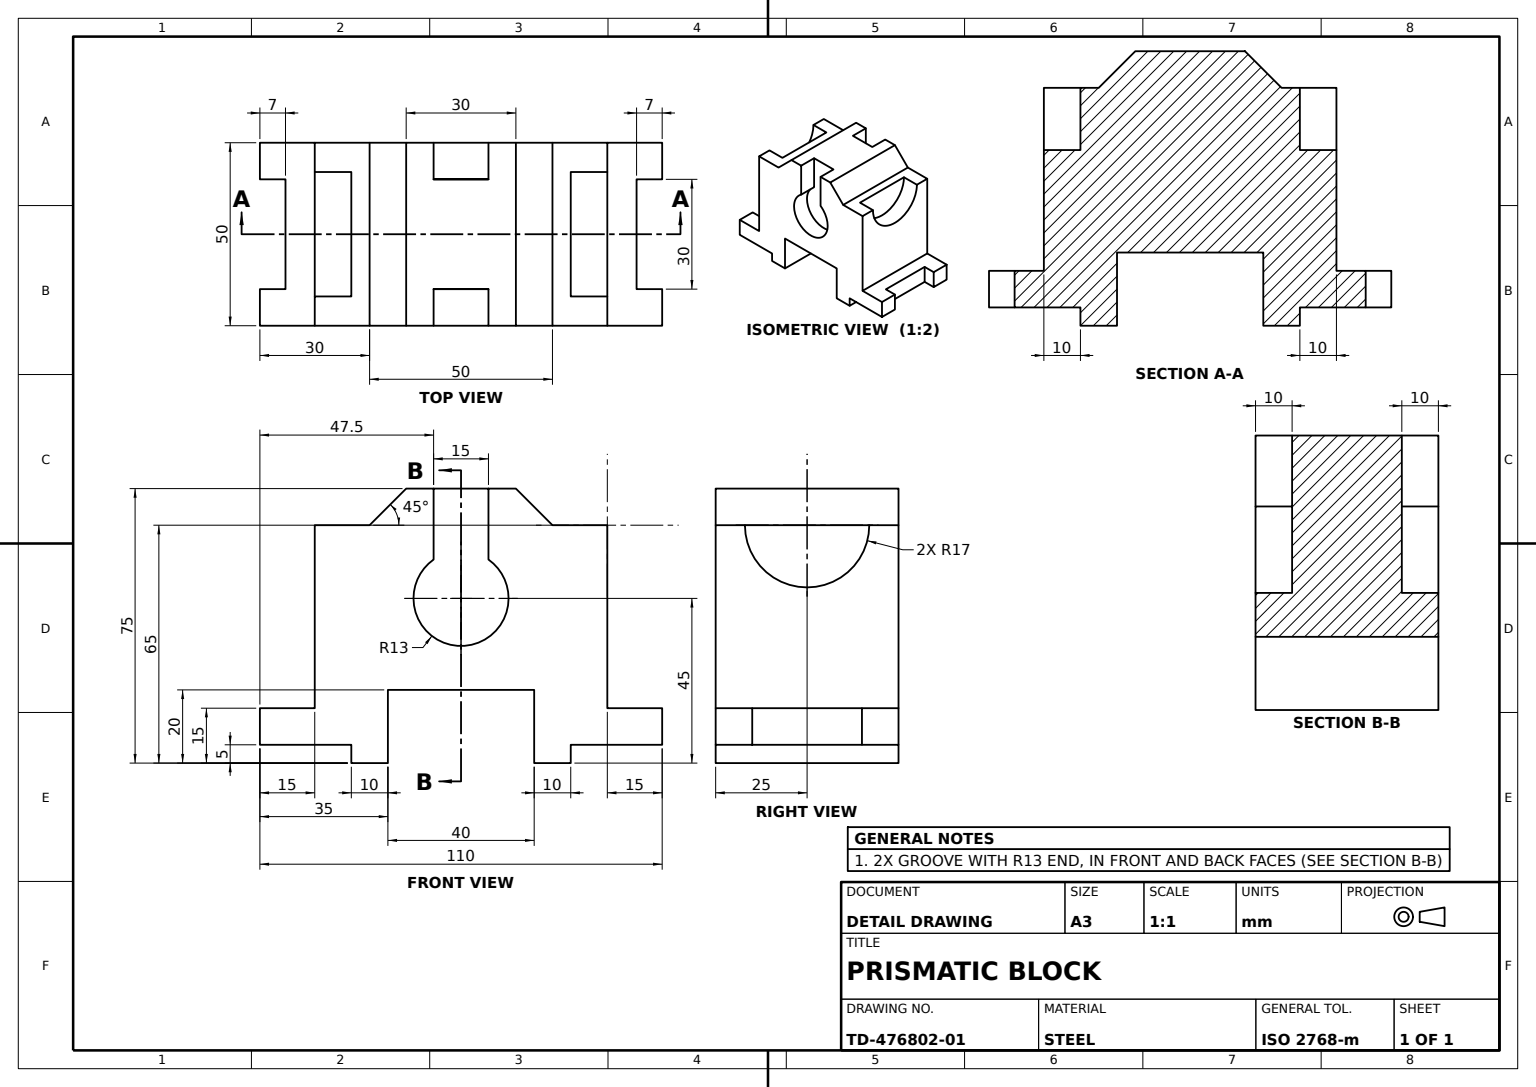
ISO-10303-21;
HEADER;
FILE_DESCRIPTION((''),'2;1');
FILE_NAME('','',(''),(''),'','','');
FILE_SCHEMA(('AUTOMOTIVE_DESIGN'));
ENDSEC;
DATA;
#1=APPLICATION_CONTEXT('');
#2=PRODUCT_CONTEXT('',#1,'mechanical');
#3=PRODUCT('','','',(#2));
#4=PRODUCT_DEFINITION_FORMATION('','',#3);
#5=PRODUCT_DEFINITION_CONTEXT('',#1,'design');
#6=PRODUCT_DEFINITION('','',#4,#5);
#7=PRODUCT_DEFINITION_SHAPE('','',#6);
#8=(LENGTH_UNIT()NAMED_UNIT(*)SI_UNIT(.MILLI.,.METRE.));
#9=(NAMED_UNIT(*)PLANE_ANGLE_UNIT()SI_UNIT($,.RADIAN.));
#10=(NAMED_UNIT(*)SI_UNIT($,.STERADIAN.)SOLID_ANGLE_UNIT());
#11=UNCERTAINTY_MEASURE_WITH_UNIT(LENGTH_MEASURE(1.E-05),#8,'distance_accuracy_value','');
#12=(GEOMETRIC_REPRESENTATION_CONTEXT(3)GLOBAL_UNCERTAINTY_ASSIGNED_CONTEXT((#11))GLOBAL_UNIT_ASSIGNED_CONTEXT((#8,#9,#10))REPRESENTATION_CONTEXT('',''));
#13=CARTESIAN_POINT('',(22.5,55.61838,0.));
#14=VERTEX_POINT('',#13);
#15=CARTESIAN_POINT('',(22.5,75.,0.));
#16=VERTEX_POINT('',#15);
#17=DIRECTION('',(0.,1.,0.));
#18=VECTOR('',#17,1000.);
#19=LINE('',#15,#18);
#20=EDGE_CURVE('',#14,#16,#19,.T.);
#21=ORIENTED_EDGE('',*,*,#20,.T.);
#22=CARTESIAN_POINT('',(22.5,75.,10.));
#23=VERTEX_POINT('',#22);
#24=DIRECTION('',(0.,0.,-1.));
#25=VECTOR('',#24,1000.);
#26=LINE('',#22,#25);
#27=EDGE_CURVE('',#23,#16,#26,.T.);
#28=ORIENTED_EDGE('',*,*,#27,.F.);
#29=CARTESIAN_POINT('',(22.5,55.61838,10.));
#30=VERTEX_POINT('',#29);
#31=LINE('',#22,#18);
#32=EDGE_CURVE('',#30,#23,#31,.T.);
#33=ORIENTED_EDGE('',*,*,#32,.F.);
#34=LINE('',#29,#25);
#35=EDGE_CURVE('',#30,#14,#34,.T.);
#36=ORIENTED_EDGE('',*,*,#35,.T.);
#37=EDGE_LOOP('',(#21,#28,#33,#36));
#38=FACE_OUTER_BOUND('',#37,.T.);
#39=DIRECTION('',(-1.,0.,0.));
#40=DIRECTION('',(0.,0.,1.));
#41=AXIS2_PLACEMENT_3D('',#22,#39,#40);
#42=PLANE('',#41);
#43=ADVANCED_FACE('',(#38),#42,.F.);
#44=CARTESIAN_POINT('',(0.,65.,8.));
#45=VERTEX_POINT('',#44);
#46=CARTESIAN_POINT('',(0.,65.,42.));
#47=VERTEX_POINT('',#46);
#48=CARTESIAN_POINT('',(0.,65.,25.));
#49=AXIS2_PLACEMENT_3D('',#48,#39,#40);
#50=CIRCLE('',#49,17.);
#51=EDGE_CURVE('',#45,#47,#50,.T.);
#52=ORIENTED_EDGE('',*,*,#51,.T.);
#53=LINE('',#44,#25);
#54=EDGE_CURVE('',#47,#45,#53,.T.);
#55=ORIENTED_EDGE('',*,*,#54,.T.);
#56=EDGE_LOOP('',(#52,#55));
#57=FACE_OUTER_BOUND('',#56,.T.);
#58=PLANE('',#49);
#59=ADVANCED_FACE('',(#57),#58,.T.);
#60=CARTESIAN_POINT('',(22.5,75.,50.));
#61=VERTEX_POINT('',#60);
#62=CARTESIAN_POINT('',(22.5,55.61838,50.));
#63=VERTEX_POINT('',#62);
#64=DIRECTION('',(0.,-1.,0.));
#65=VECTOR('',#64,1000.);
#66=LINE('',#60,#65);
#67=EDGE_CURVE('',#61,#63,#66,.T.);
#68=ORIENTED_EDGE('',*,*,#67,.T.);
#69=CARTESIAN_POINT('',(22.5,55.61838,40.));
#70=VERTEX_POINT('',#69);
#71=VECTOR('',#40,1000.);
#72=LINE('',#69,#71);
#73=EDGE_CURVE('',#70,#63,#72,.T.);
#74=ORIENTED_EDGE('',*,*,#73,.F.);
#75=CARTESIAN_POINT('',(22.5,75.,40.));
#76=VERTEX_POINT('',#75);
#77=LINE('',#75,#65);
#78=EDGE_CURVE('',#76,#70,#77,.T.);
#79=ORIENTED_EDGE('',*,*,#78,.F.);
#80=LINE('',#75,#71);
#81=EDGE_CURVE('',#76,#61,#80,.T.);
#82=ORIENTED_EDGE('',*,*,#81,.T.);
#83=EDGE_LOOP('',(#68,#74,#79,#82));
#84=FACE_OUTER_BOUND('',#83,.T.);
#85=AXIS2_PLACEMENT_3D('',#75,#39,#40);
#86=PLANE('',#85);
#87=ADVANCED_FACE('',(#84),#86,.F.);
#88=CARTESIAN_POINT('',(85.,5.,40.));
#89=VERTEX_POINT('',#88);
#90=CARTESIAN_POINT('',(85.,15.,40.));
#91=VERTEX_POINT('',#90);
#92=LINE('',#88,#18);
#93=EDGE_CURVE('',#89,#91,#92,.T.);
#94=ORIENTED_EDGE('',*,*,#93,.F.);
#95=CARTESIAN_POINT('',(78.,5.,40.));
#96=VERTEX_POINT('',#95);
#97=DIRECTION('',(1.,0.,0.));
#98=VECTOR('',#97,1000.);
#99=LINE('',#95,#98);
#100=EDGE_CURVE('',#96,#89,#99,.T.);
#101=ORIENTED_EDGE('',*,*,#100,.F.);
#102=CARTESIAN_POINT('',(78.,15.,40.));
#103=VERTEX_POINT('',#102);
#104=LINE('',#95,#18);
#105=EDGE_CURVE('',#96,#103,#104,.T.);
#106=ORIENTED_EDGE('',*,*,#105,.T.);
#107=LINE('',#102,#98);
#108=EDGE_CURVE('',#103,#91,#107,.T.);
#109=ORIENTED_EDGE('',*,*,#108,.T.);
#110=EDGE_LOOP('',(#94,#101,#106,#109));
#111=FACE_OUTER_BOUND('',#110,.T.);
#112=AXIS2_PLACEMENT_3D('',#95,#40,#97);
#113=PLANE('',#112);
#114=ADVANCED_FACE('',(#111),#113,.F.);
#115=CARTESIAN_POINT('',(-10.,65.,8.));
#116=VERTEX_POINT('',#115);
#117=CARTESIAN_POINT('',(-10.,65.,42.));
#118=VERTEX_POINT('',#117);
#119=CARTESIAN_POINT('',(-10.,65.,25.));
#120=AXIS2_PLACEMENT_3D('',#119,#39,#40);
#121=CIRCLE('',#120,17.);
#122=EDGE_CURVE('',#116,#118,#121,.T.);
#123=ORIENTED_EDGE('',*,*,#122,.T.);
#124=VECTOR('',#39,1000.);
#125=LINE('',#46,#124);
#126=EDGE_CURVE('',#47,#118,#125,.T.);
#127=ORIENTED_EDGE('',*,*,#126,.F.);
#128=ORIENTED_EDGE('',*,*,#51,.F.);
#129=LINE('',#44,#124);
#130=EDGE_CURVE('',#45,#116,#129,.T.);
#131=ORIENTED_EDGE('',*,*,#130,.T.);
#132=EDGE_LOOP('',(#123,#127,#128,#131));
#133=FACE_OUTER_BOUND('',#132,.T.);
#134=CYLINDRICAL_SURFACE('',#49,17.);
#135=ADVANCED_FACE('',(#133),#134,.F.);
#136=CARTESIAN_POINT('',(55.,65.,50.));
#137=VERTEX_POINT('',#136);
#138=CARTESIAN_POINT('',(45.,75.,50.));
#139=VERTEX_POINT('',#138);
#140=DIRECTION('',(-0.707106781,0.707106781,0.));
#141=VECTOR('',#140,1000.);
#142=LINE('',#138,#141);
#143=EDGE_CURVE('',#137,#139,#142,.T.);
#144=ORIENTED_EDGE('',*,*,#143,.F.);
#145=CARTESIAN_POINT('',(55.,65.,0.));
#146=VERTEX_POINT('',#145);
#147=LINE('',#136,#25);
#148=EDGE_CURVE('',#137,#146,#147,.T.);
#149=ORIENTED_EDGE('',*,*,#148,.T.);
#150=CARTESIAN_POINT('',(45.,75.,0.));
#151=VERTEX_POINT('',#150);
#152=LINE('',#150,#141);
#153=EDGE_CURVE('',#146,#151,#152,.T.);
#154=ORIENTED_EDGE('',*,*,#153,.T.);
#155=LINE('',#138,#25);
#156=EDGE_CURVE('',#139,#151,#155,.T.);
#157=ORIENTED_EDGE('',*,*,#156,.F.);
#158=EDGE_LOOP('',(#144,#149,#154,#157));
#159=FACE_OUTER_BOUND('',#158,.T.);
#160=DIRECTION('',(-0.707106781,-0.707106781,0.));
#161=DIRECTION('',(0.707106781,-0.707106781,0.));
#162=AXIS2_PLACEMENT_3D('',#138,#160,#161);
#163=PLANE('',#162);
#164=ADVANCED_FACE('',(#159),#163,.F.);
#165=CARTESIAN_POINT('',(60.,65.,42.));
#166=VERTEX_POINT('',#165);
#167=CARTESIAN_POINT('',(60.,65.,8.));
#168=VERTEX_POINT('',#167);
#169=CARTESIAN_POINT('',(60.,65.,25.));
#170=AXIS2_PLACEMENT_3D('',#169,#97,#24);
#171=CIRCLE('',#170,17.);
#172=EDGE_CURVE('',#166,#168,#171,.T.);
#173=ORIENTED_EDGE('',*,*,#172,.T.);
#174=LINE('',#165,#71);
#175=EDGE_CURVE('',#168,#166,#174,.T.);
#176=ORIENTED_EDGE('',*,*,#175,.T.);
#177=EDGE_LOOP('',(#173,#176));
#178=FACE_OUTER_BOUND('',#177,.T.);
#179=PLANE('',#170);
#180=ADVANCED_FACE('',(#178),#179,.T.);
#181=CARTESIAN_POINT('',(0.,0.,50.));
#182=VERTEX_POINT('',#181);
#183=CARTESIAN_POINT('',(0.,0.,0.));
#184=VERTEX_POINT('',#183);
#185=LINE('',#181,#25);
#186=EDGE_CURVE('',#182,#184,#185,.T.);
#187=ORIENTED_EDGE('',*,*,#186,.T.);
#188=CARTESIAN_POINT('',(10.,0.,0.));
#189=VERTEX_POINT('',#188);
#190=LINE('',#183,#98);
#191=EDGE_CURVE('',#184,#189,#190,.T.);
#192=ORIENTED_EDGE('',*,*,#191,.T.);
#193=CARTESIAN_POINT('',(10.,0.,50.));
#194=VERTEX_POINT('',#193);
#195=LINE('',#193,#25);
#196=EDGE_CURVE('',#194,#189,#195,.T.);
#197=ORIENTED_EDGE('',*,*,#196,.F.);
#198=LINE('',#181,#98);
#199=EDGE_CURVE('',#182,#194,#198,.T.);
#200=ORIENTED_EDGE('',*,*,#199,.F.);
#201=EDGE_LOOP('',(#187,#192,#197,#200));
#202=FACE_OUTER_BOUND('',#201,.T.);
#203=AXIS2_PLACEMENT_3D('',#181,#17,#40);
#204=PLANE('',#203);
#205=ADVANCED_FACE('',(#202),#204,.F.);
#206=CARTESIAN_POINT('',(37.5,75.,10.));
#207=VERTEX_POINT('',#206);
#208=CARTESIAN_POINT('',(30.,75.,10.));
#209=LINE('',#208,#98);
#210=EDGE_CURVE('',#23,#207,#209,.T.);
#211=ORIENTED_EDGE('',*,*,#210,.T.);
#212=CARTESIAN_POINT('',(37.5,55.61838,10.));
#213=VERTEX_POINT('',#212);
#214=LINE('',#206,#65);
#215=EDGE_CURVE('',#207,#213,#214,.T.);
#216=ORIENTED_EDGE('',*,*,#215,.T.);
#217=CARTESIAN_POINT('',(43.,45.,10.));
#218=VERTEX_POINT('',#217);
#219=CARTESIAN_POINT('',(30.,45.,10.));
#220=AXIS2_PLACEMENT_3D('',#219,#24,#39);
#221=CIRCLE('',#220,13.);
#222=EDGE_CURVE('',#213,#218,#221,.T.);
#223=ORIENTED_EDGE('',*,*,#222,.T.);
#224=CARTESIAN_POINT('',(17.,45.,10.));
#225=VERTEX_POINT('',#224);
#226=EDGE_CURVE('',#218,#225,#221,.T.);
#227=ORIENTED_EDGE('',*,*,#226,.T.);
#228=EDGE_CURVE('',#225,#30,#221,.T.);
#229=ORIENTED_EDGE('',*,*,#228,.T.);
#230=ORIENTED_EDGE('',*,*,#32,.T.);
#231=EDGE_LOOP('',(#211,#216,#223,#227,#229,#230));
#232=FACE_OUTER_BOUND('',#231,.T.);
#233=PLANE('',#220);
#234=ADVANCED_FACE('',(#232),#233,.T.);
#235=CARTESIAN_POINT('',(17.,45.,0.));
#236=VERTEX_POINT('',#235);
#237=CARTESIAN_POINT('',(30.,45.,0.));
#238=AXIS2_PLACEMENT_3D('',#237,#24,#39);
#239=CIRCLE('',#238,13.);
#240=EDGE_CURVE('',#236,#14,#239,.T.);
#241=ORIENTED_EDGE('',*,*,#240,.T.);
#242=ORIENTED_EDGE('',*,*,#35,.F.);
#243=ORIENTED_EDGE('',*,*,#228,.F.);
#244=LINE('',#224,#25);
#245=EDGE_CURVE('',#225,#236,#244,.T.);
#246=ORIENTED_EDGE('',*,*,#245,.T.);
#247=EDGE_LOOP('',(#241,#242,#243,#246));
#248=FACE_OUTER_BOUND('',#247,.T.);
#249=CYLINDRICAL_SURFACE('',#220,13.);
#250=ADVANCED_FACE('',(#248),#249,.F.);
#251=CARTESIAN_POINT('',(15.,75.,50.));
#252=VERTEX_POINT('',#251);
#253=CARTESIAN_POINT('',(5.,65.,50.));
#254=VERTEX_POINT('',#253);
#255=VECTOR('',#160,1000.);
#256=LINE('',#251,#255);
#257=EDGE_CURVE('',#252,#254,#256,.T.);
#258=ORIENTED_EDGE('',*,*,#257,.F.);
#259=CARTESIAN_POINT('',(15.,75.,0.));
#260=VERTEX_POINT('',#259);
#261=LINE('',#251,#25);
#262=EDGE_CURVE('',#252,#260,#261,.T.);
#263=ORIENTED_EDGE('',*,*,#262,.T.);
#264=CARTESIAN_POINT('',(5.,65.,0.));
#265=VERTEX_POINT('',#264);
#266=LINE('',#259,#255);
#267=EDGE_CURVE('',#260,#265,#266,.T.);
#268=ORIENTED_EDGE('',*,*,#267,.T.);
#269=LINE('',#253,#25);
#270=EDGE_CURVE('',#254,#265,#269,.T.);
#271=ORIENTED_EDGE('',*,*,#270,.F.);
#272=EDGE_LOOP('',(#258,#263,#268,#271));
#273=FACE_OUTER_BOUND('',#272,.T.);
#274=DIRECTION('',(0.707106781,0.707106781,0.));
#275=AXIS2_PLACEMENT_3D('',#251,#161,#274);
#276=PLANE('',#275);
#277=ADVANCED_FACE('',(#273),#276,.F.);
#278=CARTESIAN_POINT('',(50.,20.,50.));
#279=VERTEX_POINT('',#278);
#280=CARTESIAN_POINT('',(50.,20.,0.));
#281=VERTEX_POINT('',#280);
#282=LINE('',#278,#25);
#283=EDGE_CURVE('',#279,#281,#282,.T.);
#284=ORIENTED_EDGE('',*,*,#283,.F.);
#285=CARTESIAN_POINT('',(10.,20.,50.));
#286=VERTEX_POINT('',#285);
#287=LINE('',#285,#98);
#288=EDGE_CURVE('',#286,#279,#287,.T.);
#289=ORIENTED_EDGE('',*,*,#288,.F.);
#290=CARTESIAN_POINT('',(10.,20.,0.));
#291=VERTEX_POINT('',#290);
#292=LINE('',#285,#25);
#293=EDGE_CURVE('',#286,#291,#292,.T.);
#294=ORIENTED_EDGE('',*,*,#293,.T.);
#295=LINE('',#290,#98);
#296=EDGE_CURVE('',#291,#281,#295,.T.);
#297=ORIENTED_EDGE('',*,*,#296,.T.);
#298=EDGE_LOOP('',(#284,#289,#294,#297));
#299=FACE_OUTER_BOUND('',#298,.T.);
#300=AXIS2_PLACEMENT_3D('',#285,#17,#40);
#301=PLANE('',#300);
#302=ADVANCED_FACE('',(#299),#301,.F.);
#303=CARTESIAN_POINT('',(78.,5.,10.));
#304=VERTEX_POINT('',#303);
#305=CARTESIAN_POINT('',(78.,15.,10.));
#306=VERTEX_POINT('',#305);
#307=LINE('',#303,#18);
#308=EDGE_CURVE('',#304,#306,#307,.T.);
#309=ORIENTED_EDGE('',*,*,#308,.T.);
#310=LINE('',#305,#71);
#311=EDGE_CURVE('',#306,#103,#310,.T.);
#312=ORIENTED_EDGE('',*,*,#311,.T.);
#313=ORIENTED_EDGE('',*,*,#105,.F.);
#314=LINE('',#303,#71);
#315=EDGE_CURVE('',#304,#96,#314,.T.);
#316=ORIENTED_EDGE('',*,*,#315,.F.);
#317=EDGE_LOOP('',(#309,#312,#313,#316));
#318=FACE_OUTER_BOUND('',#317,.T.);
#319=AXIS2_PLACEMENT_3D('',#303,#39,#40);
#320=PLANE('',#319);
#321=ADVANCED_FACE('',(#318),#320,.F.);
#322=CARTESIAN_POINT('',(50.,0.,0.));
#323=VERTEX_POINT('',#322);
#324=LINE('',#280,#65);
#325=EDGE_CURVE('',#281,#323,#324,.T.);
#326=ORIENTED_EDGE('',*,*,#325,.T.);
#327=CARTESIAN_POINT('',(50.,0.,50.));
#328=VERTEX_POINT('',#327);
#329=LINE('',#327,#25);
#330=EDGE_CURVE('',#328,#323,#329,.T.);
#331=ORIENTED_EDGE('',*,*,#330,.F.);
#332=LINE('',#278,#65);
#333=EDGE_CURVE('',#279,#328,#332,.T.);
#334=ORIENTED_EDGE('',*,*,#333,.F.);
#335=ORIENTED_EDGE('',*,*,#283,.T.);
#336=EDGE_LOOP('',(#326,#331,#334,#335));
#337=FACE_OUTER_BOUND('',#336,.T.);
#338=AXIS2_PLACEMENT_3D('',#278,#97,#24);
#339=PLANE('',#338);
#340=ADVANCED_FACE('',(#337),#339,.F.);
#341=CARTESIAN_POINT('',(-18.,5.,10.));
#342=VERTEX_POINT('',#341);
#343=CARTESIAN_POINT('',(-25.,5.,10.));
#344=VERTEX_POINT('',#343);
#345=LINE('',#341,#124);
#346=EDGE_CURVE('',#342,#344,#345,.T.);
#347=ORIENTED_EDGE('',*,*,#346,.F.);
#348=CARTESIAN_POINT('',(-18.,15.,10.));
#349=VERTEX_POINT('',#348);
#350=LINE('',#341,#18);
#351=EDGE_CURVE('',#342,#349,#350,.T.);
#352=ORIENTED_EDGE('',*,*,#351,.T.);
#353=CARTESIAN_POINT('',(-25.,15.,10.));
#354=VERTEX_POINT('',#353);
#355=LINE('',#348,#124);
#356=EDGE_CURVE('',#349,#354,#355,.T.);
#357=ORIENTED_EDGE('',*,*,#356,.T.);
#358=LINE('',#343,#18);
#359=EDGE_CURVE('',#344,#354,#358,.T.);
#360=ORIENTED_EDGE('',*,*,#359,.F.);
#361=EDGE_LOOP('',(#347,#352,#357,#360));
#362=FACE_OUTER_BOUND('',#361,.T.);
#363=AXIS2_PLACEMENT_3D('',#341,#24,#39);
#364=PLANE('',#363);
#365=ADVANCED_FACE('',(#362),#364,.F.);
#366=ORIENTED_EDGE('',*,*,#186,.F.);
#367=CARTESIAN_POINT('',(0.,5.,50.));
#368=VERTEX_POINT('',#367);
#369=LINE('',#181,#65);
#370=EDGE_CURVE('',#368,#182,#369,.T.);
#371=ORIENTED_EDGE('',*,*,#370,.F.);
#372=CARTESIAN_POINT('',(0.,5.,0.));
#373=VERTEX_POINT('',#372);
#374=LINE('',#367,#25);
#375=EDGE_CURVE('',#368,#373,#374,.T.);
#376=ORIENTED_EDGE('',*,*,#375,.T.);
#377=LINE('',#183,#65);
#378=EDGE_CURVE('',#373,#184,#377,.T.);
#379=ORIENTED_EDGE('',*,*,#378,.T.);
#380=EDGE_LOOP('',(#366,#371,#376,#379));
#381=FACE_OUTER_BOUND('',#380,.T.);
#382=AXIS2_PLACEMENT_3D('',#181,#97,#24);
#383=PLANE('',#382);
#384=ADVANCED_FACE('',(#381),#383,.F.);
#385=CARTESIAN_POINT('',(17.,45.,40.));
#386=VERTEX_POINT('',#385);
#387=CARTESIAN_POINT('',(17.,45.,50.));
#388=VERTEX_POINT('',#387);
#389=LINE('',#385,#71);
#390=EDGE_CURVE('',#386,#388,#389,.T.);
#391=ORIENTED_EDGE('',*,*,#390,.F.);
#392=CARTESIAN_POINT('',(30.,45.,40.));
#393=AXIS2_PLACEMENT_3D('',#392,#40,#97);
#394=CIRCLE('',#393,13.);
#395=EDGE_CURVE('',#70,#386,#394,.T.);
#396=ORIENTED_EDGE('',*,*,#395,.F.);
#397=ORIENTED_EDGE('',*,*,#73,.T.);
#398=CARTESIAN_POINT('',(30.,45.,50.));
#399=AXIS2_PLACEMENT_3D('',#398,#40,#97);
#400=CIRCLE('',#399,13.);
#401=EDGE_CURVE('',#63,#388,#400,.T.);
#402=ORIENTED_EDGE('',*,*,#401,.T.);
#403=EDGE_LOOP('',(#391,#396,#397,#402));
#404=FACE_OUTER_BOUND('',#403,.T.);
#405=CYLINDRICAL_SURFACE('',#393,13.);
#406=ADVANCED_FACE('',(#404),#405,.F.);
#407=CARTESIAN_POINT('',(-25.,5.,40.));
#408=VERTEX_POINT('',#407);
#409=CARTESIAN_POINT('',(-18.,5.,40.));
#410=VERTEX_POINT('',#409);
#411=LINE('',#407,#98);
#412=EDGE_CURVE('',#408,#410,#411,.T.);
#413=ORIENTED_EDGE('',*,*,#412,.T.);
#414=LINE('',#409,#25);
#415=EDGE_CURVE('',#410,#342,#414,.T.);
#416=ORIENTED_EDGE('',*,*,#415,.T.);
#417=ORIENTED_EDGE('',*,*,#346,.T.);
#418=CARTESIAN_POINT('',(-25.,5.,0.));
#419=VERTEX_POINT('',#418);
#420=CARTESIAN_POINT('',(-25.,5.,50.));
#421=LINE('',#420,#25);
#422=EDGE_CURVE('',#344,#419,#421,.T.);
#423=ORIENTED_EDGE('',*,*,#422,.T.);
#424=LINE('',#372,#98);
#425=EDGE_CURVE('',#419,#373,#424,.T.);
#426=ORIENTED_EDGE('',*,*,#425,.T.);
#427=ORIENTED_EDGE('',*,*,#375,.F.);
#428=VERTEX_POINT('',#420);
#429=LINE('',#367,#98);
#430=EDGE_CURVE('',#428,#368,#429,.T.);
#431=ORIENTED_EDGE('',*,*,#430,.F.);
#432=EDGE_CURVE('',#428,#408,#421,.T.);
#433=ORIENTED_EDGE('',*,*,#432,.T.);
#434=EDGE_LOOP('',(#413,#416,#417,#423,#426,#427,#431,#433));
#435=FACE_OUTER_BOUND('',#434,.T.);
#436=AXIS2_PLACEMENT_3D('',#367,#17,#40);
#437=PLANE('',#436);
#438=ADVANCED_FACE('',(#435),#437,.F.);
#439=ORIENTED_EDGE('',*,*,#315,.T.);
#440=ORIENTED_EDGE('',*,*,#100,.T.);
#441=CARTESIAN_POINT('',(85.,5.,50.));
#442=VERTEX_POINT('',#441);
#443=LINE('',#441,#25);
#444=EDGE_CURVE('',#442,#89,#443,.T.);
#445=ORIENTED_EDGE('',*,*,#444,.F.);
#446=CARTESIAN_POINT('',(60.,5.,50.));
#447=VERTEX_POINT('',#446);
#448=LINE('',#446,#98);
#449=EDGE_CURVE('',#447,#442,#448,.T.);
#450=ORIENTED_EDGE('',*,*,#449,.F.);
#451=CARTESIAN_POINT('',(60.,5.,0.));
#452=VERTEX_POINT('',#451);
#453=LINE('',#446,#25);
#454=EDGE_CURVE('',#447,#452,#453,.T.);
#455=ORIENTED_EDGE('',*,*,#454,.T.);
#456=CARTESIAN_POINT('',(85.,5.,0.));
#457=VERTEX_POINT('',#456);
#458=LINE('',#451,#98);
#459=EDGE_CURVE('',#452,#457,#458,.T.);
#460=ORIENTED_EDGE('',*,*,#459,.T.);
#461=CARTESIAN_POINT('',(85.,5.,10.));
#462=VERTEX_POINT('',#461);
#463=EDGE_CURVE('',#462,#457,#443,.T.);
#464=ORIENTED_EDGE('',*,*,#463,.F.);
#465=LINE('',#461,#124);
#466=EDGE_CURVE('',#462,#304,#465,.T.);
#467=ORIENTED_EDGE('',*,*,#466,.T.);
#468=EDGE_LOOP('',(#439,#440,#445,#450,#455,#460,#464,#467));
#469=FACE_OUTER_BOUND('',#468,.T.);
#470=AXIS2_PLACEMENT_3D('',#446,#17,#40);
#471=PLANE('',#470);
#472=ADVANCED_FACE('',(#469),#471,.F.);
#473=CARTESIAN_POINT('',(37.5,55.61838,40.));
#474=VERTEX_POINT('',#473);
#475=CARTESIAN_POINT('',(37.5,75.,40.));
#476=VERTEX_POINT('',#475);
#477=LINE('',#475,#18);
#478=EDGE_CURVE('',#474,#476,#477,.T.);
#479=ORIENTED_EDGE('',*,*,#478,.F.);
#480=CARTESIAN_POINT('',(37.5,55.61838,50.));
#481=VERTEX_POINT('',#480);
#482=LINE('',#473,#71);
#483=EDGE_CURVE('',#474,#481,#482,.T.);
#484=ORIENTED_EDGE('',*,*,#483,.T.);
#485=CARTESIAN_POINT('',(37.5,75.,50.));
#486=VERTEX_POINT('',#485);
#487=LINE('',#485,#18);
#488=EDGE_CURVE('',#481,#486,#487,.T.);
#489=ORIENTED_EDGE('',*,*,#488,.T.);
#490=LINE('',#475,#71);
#491=EDGE_CURVE('',#476,#486,#490,.T.);
#492=ORIENTED_EDGE('',*,*,#491,.F.);
#493=EDGE_LOOP('',(#479,#484,#489,#492));
#494=FACE_OUTER_BOUND('',#493,.T.);
#495=AXIS2_PLACEMENT_3D('',#475,#97,#24);
#496=PLANE('',#495);
#497=ADVANCED_FACE('',(#494),#496,.F.);
#498=CARTESIAN_POINT('',(43.,45.,50.));
#499=VERTEX_POINT('',#498);
#500=EDGE_CURVE('',#499,#481,#400,.T.);
#501=ORIENTED_EDGE('',*,*,#500,.T.);
#502=ORIENTED_EDGE('',*,*,#483,.F.);
#503=CARTESIAN_POINT('',(43.,45.,40.));
#504=VERTEX_POINT('',#503);
#505=EDGE_CURVE('',#504,#474,#394,.T.);
#506=ORIENTED_EDGE('',*,*,#505,.F.);
#507=LINE('',#503,#71);
#508=EDGE_CURVE('',#504,#499,#507,.T.);
#509=ORIENTED_EDGE('',*,*,#508,.T.);
#510=EDGE_LOOP('',(#501,#502,#506,#509));
#511=FACE_OUTER_BOUND('',#510,.T.);
#512=ADVANCED_FACE('',(#511),#405,.F.);
#513=CARTESIAN_POINT('',(70.,65.,50.));
#514=VERTEX_POINT('',#513);
#515=CARTESIAN_POINT('',(70.,65.,42.));
#516=VERTEX_POINT('',#515);
#517=LINE('',#513,#25);
#518=EDGE_CURVE('',#514,#516,#517,.T.);
#519=ORIENTED_EDGE('',*,*,#518,.F.);
#520=CARTESIAN_POINT('',(70.,15.,50.));
#521=VERTEX_POINT('',#520);
#522=LINE('',#520,#18);
#523=EDGE_CURVE('',#521,#514,#522,.T.);
#524=ORIENTED_EDGE('',*,*,#523,.F.);
#525=CARTESIAN_POINT('',(70.,15.,0.));
#526=VERTEX_POINT('',#525);
#527=LINE('',#520,#25);
#528=EDGE_CURVE('',#521,#526,#527,.T.);
#529=ORIENTED_EDGE('',*,*,#528,.T.);
#530=CARTESIAN_POINT('',(70.,65.,0.));
#531=VERTEX_POINT('',#530);
#532=LINE('',#525,#18);
#533=EDGE_CURVE('',#526,#531,#532,.T.);
#534=ORIENTED_EDGE('',*,*,#533,.T.);
#535=CARTESIAN_POINT('',(70.,65.,8.));
#536=VERTEX_POINT('',#535);
#537=EDGE_CURVE('',#536,#531,#517,.T.);
#538=ORIENTED_EDGE('',*,*,#537,.F.);
#539=CARTESIAN_POINT('',(70.,65.,25.));
#540=AXIS2_PLACEMENT_3D('',#539,#97,#24);
#541=CIRCLE('',#540,17.);
#542=EDGE_CURVE('',#516,#536,#541,.T.);
#543=ORIENTED_EDGE('',*,*,#542,.F.);
#544=EDGE_LOOP('',(#519,#524,#529,#534,#538,#543));
#545=FACE_OUTER_BOUND('',#544,.T.);
#546=AXIS2_PLACEMENT_3D('',#520,#39,#40);
#547=PLANE('',#546);
#548=ADVANCED_FACE('',(#545),#547,.F.);
#549=ORIENTED_EDGE('',*,*,#226,.F.);
#550=CARTESIAN_POINT('',(43.,45.,0.));
#551=VERTEX_POINT('',#550);
#552=LINE('',#217,#25);
#553=EDGE_CURVE('',#218,#551,#552,.T.);
#554=ORIENTED_EDGE('',*,*,#553,.T.);
#555=EDGE_CURVE('',#551,#236,#239,.T.);
#556=ORIENTED_EDGE('',*,*,#555,.T.);
#557=ORIENTED_EDGE('',*,*,#245,.F.);
#558=EDGE_LOOP('',(#549,#554,#556,#557));
#559=FACE_OUTER_BOUND('',#558,.T.);
#560=ADVANCED_FACE('',(#559),#249,.F.);
#561=CARTESIAN_POINT('',(37.5,55.61838,0.));
#562=VERTEX_POINT('',#561);
#563=LINE('',#212,#25);
#564=EDGE_CURVE('',#213,#562,#563,.T.);
#565=ORIENTED_EDGE('',*,*,#564,.F.);
#566=ORIENTED_EDGE('',*,*,#215,.F.);
#567=CARTESIAN_POINT('',(37.5,75.,0.));
#568=VERTEX_POINT('',#567);
#569=LINE('',#206,#25);
#570=EDGE_CURVE('',#207,#568,#569,.T.);
#571=ORIENTED_EDGE('',*,*,#570,.T.);
#572=LINE('',#567,#65);
#573=EDGE_CURVE('',#568,#562,#572,.T.);
#574=ORIENTED_EDGE('',*,*,#573,.T.);
#575=EDGE_LOOP('',(#565,#566,#571,#574));
#576=FACE_OUTER_BOUND('',#575,.T.);
#577=AXIS2_PLACEMENT_3D('',#206,#97,#24);
#578=PLANE('',#577);
#579=ADVANCED_FACE('',(#576),#578,.F.);
#580=CARTESIAN_POINT('',(-10.,65.,0.));
#581=VERTEX_POINT('',#580);
#582=CARTESIAN_POINT('',(-10.,65.,50.));
#583=LINE('',#582,#25);
#584=EDGE_CURVE('',#116,#581,#583,.T.);
#585=ORIENTED_EDGE('',*,*,#584,.F.);
#586=ORIENTED_EDGE('',*,*,#130,.F.);
#587=ORIENTED_EDGE('',*,*,#54,.F.);
#588=ORIENTED_EDGE('',*,*,#126,.T.);
#589=VERTEX_POINT('',#582);
#590=EDGE_CURVE('',#589,#118,#583,.T.);
#591=ORIENTED_EDGE('',*,*,#590,.F.);
#592=LINE('',#582,#124);
#593=EDGE_CURVE('',#254,#589,#592,.T.);
#594=ORIENTED_EDGE('',*,*,#593,.F.);
#595=ORIENTED_EDGE('',*,*,#270,.T.);
#596=LINE('',#580,#124);
#597=EDGE_CURVE('',#265,#581,#596,.T.);
#598=ORIENTED_EDGE('',*,*,#597,.T.);
#599=EDGE_LOOP('',(#585,#586,#587,#588,#591,#594,#595,#598));
#600=FACE_OUTER_BOUND('',#599,.T.);
#601=AXIS2_PLACEMENT_3D('',#582,#64,#24);
#602=PLANE('',#601);
#603=ADVANCED_FACE('',(#600),#602,.F.);
#604=CARTESIAN_POINT('',(-25.,15.,40.));
#605=VERTEX_POINT('',#604);
#606=CARTESIAN_POINT('',(-18.,15.,40.));
#607=VERTEX_POINT('',#606);
#608=LINE('',#604,#98);
#609=EDGE_CURVE('',#605,#607,#608,.T.);
#610=ORIENTED_EDGE('',*,*,#609,.F.);
#611=CARTESIAN_POINT('',(-25.,15.,50.));
#612=VERTEX_POINT('',#611);
#613=LINE('',#611,#25);
#614=EDGE_CURVE('',#612,#605,#613,.T.);
#615=ORIENTED_EDGE('',*,*,#614,.F.);
#616=CARTESIAN_POINT('',(-10.,15.,50.));
#617=VERTEX_POINT('',#616);
#618=LINE('',#611,#124);
#619=EDGE_CURVE('',#617,#612,#618,.T.);
#620=ORIENTED_EDGE('',*,*,#619,.F.);
#621=CARTESIAN_POINT('',(-10.,15.,0.));
#622=VERTEX_POINT('',#621);
#623=LINE('',#616,#25);
#624=EDGE_CURVE('',#617,#622,#623,.T.);
#625=ORIENTED_EDGE('',*,*,#624,.T.);
#626=CARTESIAN_POINT('',(-25.,15.,0.));
#627=VERTEX_POINT('',#626);
#628=LINE('',#626,#124);
#629=EDGE_CURVE('',#622,#627,#628,.T.);
#630=ORIENTED_EDGE('',*,*,#629,.T.);
#631=EDGE_CURVE('',#354,#627,#613,.T.);
#632=ORIENTED_EDGE('',*,*,#631,.F.);
#633=ORIENTED_EDGE('',*,*,#356,.F.);
#634=LINE('',#606,#25);
#635=EDGE_CURVE('',#607,#349,#634,.T.);
#636=ORIENTED_EDGE('',*,*,#635,.F.);
#637=EDGE_LOOP('',(#610,#615,#620,#625,#630,#632,#633,#636));
#638=FACE_OUTER_BOUND('',#637,.T.);
#639=AXIS2_PLACEMENT_3D('',#611,#64,#24);
#640=PLANE('',#639);
#641=ADVANCED_FACE('',(#638),#640,.F.);
#642=LINE('',#420,#65);
#643=EDGE_CURVE('',#612,#428,#642,.T.);
#644=ORIENTED_EDGE('',*,*,#643,.F.);
#645=ORIENTED_EDGE('',*,*,#614,.T.);
#646=LINE('',#407,#18);
#647=EDGE_CURVE('',#408,#605,#646,.T.);
#648=ORIENTED_EDGE('',*,*,#647,.F.);
#649=ORIENTED_EDGE('',*,*,#432,.F.);
#650=EDGE_LOOP('',(#644,#645,#648,#649));
#651=FACE_OUTER_BOUND('',#650,.T.);
#652=AXIS2_PLACEMENT_3D('',#420,#97,#24);
#653=PLANE('',#652);
#654=ADVANCED_FACE('',(#651),#653,.F.);
#655=ORIENTED_EDGE('',*,*,#478,.T.);
#656=CARTESIAN_POINT('',(30.,75.,40.));
#657=LINE('',#656,#124);
#658=EDGE_CURVE('',#476,#76,#657,.T.);
#659=ORIENTED_EDGE('',*,*,#658,.T.);
#660=ORIENTED_EDGE('',*,*,#78,.T.);
#661=ORIENTED_EDGE('',*,*,#395,.T.);
#662=EDGE_CURVE('',#386,#504,#394,.T.);
#663=ORIENTED_EDGE('',*,*,#662,.T.);
#664=ORIENTED_EDGE('',*,*,#505,.T.);
#665=EDGE_LOOP('',(#655,#659,#660,#661,#663,#664));
#666=FACE_OUTER_BOUND('',#665,.T.);
#667=PLANE('',#393);
#668=ADVANCED_FACE('',(#666),#667,.T.);
#669=ORIENTED_EDGE('',*,*,#584,.T.);
#670=LINE('',#621,#65);
#671=EDGE_CURVE('',#581,#622,#670,.T.);
#672=ORIENTED_EDGE('',*,*,#671,.T.);
#673=ORIENTED_EDGE('',*,*,#624,.F.);
#674=LINE('',#616,#65);
#675=EDGE_CURVE('',#589,#617,#674,.T.);
#676=ORIENTED_EDGE('',*,*,#675,.F.);
#677=ORIENTED_EDGE('',*,*,#590,.T.);
#678=ORIENTED_EDGE('',*,*,#122,.F.);
#679=EDGE_LOOP('',(#669,#672,#673,#676,#677,#678));
#680=FACE_OUTER_BOUND('',#679,.T.);
#681=AXIS2_PLACEMENT_3D('',#616,#97,#24);
#682=PLANE('',#681);
#683=ADVANCED_FACE('',(#680),#682,.F.);
#684=ORIENTED_EDGE('',*,*,#444,.T.);
#685=ORIENTED_EDGE('',*,*,#93,.T.);
#686=CARTESIAN_POINT('',(85.,15.,50.));
#687=VERTEX_POINT('',#686);
#688=LINE('',#686,#25);
#689=EDGE_CURVE('',#687,#91,#688,.T.);
#690=ORIENTED_EDGE('',*,*,#689,.F.);
#691=LINE('',#441,#18);
#692=EDGE_CURVE('',#442,#687,#691,.T.);
#693=ORIENTED_EDGE('',*,*,#692,.F.);
#694=EDGE_LOOP('',(#684,#685,#690,#693));
#695=FACE_OUTER_BOUND('',#694,.T.);
#696=AXIS2_PLACEMENT_3D('',#441,#39,#40);
#697=PLANE('',#696);
#698=ADVANCED_FACE('',(#695),#697,.F.);
#699=ORIENTED_EDGE('',*,*,#518,.T.);
#700=LINE('',#165,#98);
#701=EDGE_CURVE('',#166,#516,#700,.T.);
#702=ORIENTED_EDGE('',*,*,#701,.F.);
#703=ORIENTED_EDGE('',*,*,#175,.F.);
#704=LINE('',#167,#98);
#705=EDGE_CURVE('',#168,#536,#704,.T.);
#706=ORIENTED_EDGE('',*,*,#705,.T.);
#707=ORIENTED_EDGE('',*,*,#537,.T.);
#708=LINE('',#530,#124);
#709=EDGE_CURVE('',#531,#146,#708,.T.);
#710=ORIENTED_EDGE('',*,*,#709,.T.);
#711=ORIENTED_EDGE('',*,*,#148,.F.);
#712=LINE('',#513,#124);
#713=EDGE_CURVE('',#514,#137,#712,.T.);
#714=ORIENTED_EDGE('',*,*,#713,.F.);
#715=EDGE_LOOP('',(#699,#702,#703,#706,#707,#710,#711,#714));
#716=FACE_OUTER_BOUND('',#715,.T.);
#717=AXIS2_PLACEMENT_3D('',#513,#64,#24);
#718=PLANE('',#717);
#719=ADVANCED_FACE('',(#716),#718,.F.);
#720=ORIENTED_EDGE('',*,*,#210,.F.);
#721=ORIENTED_EDGE('',*,*,#27,.T.);
#722=LINE('',#15,#124);
#723=EDGE_CURVE('',#16,#260,#722,.T.);
#724=ORIENTED_EDGE('',*,*,#723,.T.);
#725=ORIENTED_EDGE('',*,*,#262,.F.);
#726=LINE('',#485,#124);
#727=EDGE_CURVE('',#61,#252,#726,.T.);
#728=ORIENTED_EDGE('',*,*,#727,.F.);
#729=ORIENTED_EDGE('',*,*,#81,.F.);
#730=ORIENTED_EDGE('',*,*,#658,.F.);
#731=ORIENTED_EDGE('',*,*,#491,.T.);
#732=EDGE_CURVE('',#139,#486,#726,.T.);
#733=ORIENTED_EDGE('',*,*,#732,.F.);
#734=ORIENTED_EDGE('',*,*,#156,.T.);
#735=EDGE_CURVE('',#151,#568,#722,.T.);
#736=ORIENTED_EDGE('',*,*,#735,.T.);
#737=ORIENTED_EDGE('',*,*,#570,.F.);
#738=EDGE_LOOP('',(#720,#721,#724,#725,#728,#729,#730,#731,#733,#734,#736,#737));
#739=FACE_OUTER_BOUND('',#738,.T.);
#740=AXIS2_PLACEMENT_3D('',#60,#64,#24);
#741=PLANE('',#740);
#742=ADVANCED_FACE('',(#739),#741,.F.);
#743=CARTESIAN_POINT('',(60.,0.,50.));
#744=VERTEX_POINT('',#743);
#745=LINE('',#743,#18);
#746=EDGE_CURVE('',#744,#447,#745,.T.);
#747=ORIENTED_EDGE('',*,*,#746,.F.);
#748=CARTESIAN_POINT('',(60.,0.,0.));
#749=VERTEX_POINT('',#748);
#750=LINE('',#743,#25);
#751=EDGE_CURVE('',#744,#749,#750,.T.);
#752=ORIENTED_EDGE('',*,*,#751,.T.);
#753=LINE('',#748,#18);
#754=EDGE_CURVE('',#749,#452,#753,.T.);
#755=ORIENTED_EDGE('',*,*,#754,.T.);
#756=ORIENTED_EDGE('',*,*,#454,.F.);
#757=EDGE_LOOP('',(#747,#752,#755,#756));
#758=FACE_OUTER_BOUND('',#757,.T.);
#759=AXIS2_PLACEMENT_3D('',#743,#39,#40);
#760=PLANE('',#759);
#761=ADVANCED_FACE('',(#758),#760,.F.);
#762=ORIENTED_EDGE('',*,*,#311,.F.);
#763=CARTESIAN_POINT('',(85.,15.,10.));
#764=VERTEX_POINT('',#763);
#765=LINE('',#763,#124);
#766=EDGE_CURVE('',#764,#306,#765,.T.);
#767=ORIENTED_EDGE('',*,*,#766,.F.);
#768=CARTESIAN_POINT('',(85.,15.,0.));
#769=VERTEX_POINT('',#768);
#770=EDGE_CURVE('',#764,#769,#688,.T.);
#771=ORIENTED_EDGE('',*,*,#770,.T.);
#772=LINE('',#525,#124);
#773=EDGE_CURVE('',#769,#526,#772,.T.);
#774=ORIENTED_EDGE('',*,*,#773,.T.);
#775=ORIENTED_EDGE('',*,*,#528,.F.);
#776=LINE('',#520,#124);
#777=EDGE_CURVE('',#687,#521,#776,.T.);
#778=ORIENTED_EDGE('',*,*,#777,.F.);
#779=ORIENTED_EDGE('',*,*,#689,.T.);
#780=ORIENTED_EDGE('',*,*,#108,.F.);
#781=EDGE_LOOP('',(#762,#767,#771,#774,#775,#778,#779,#780));
#782=FACE_OUTER_BOUND('',#781,.T.);
#783=AXIS2_PLACEMENT_3D('',#520,#64,#24);
#784=PLANE('',#783);
#785=ADVANCED_FACE('',(#782),#784,.F.);
#786=ORIENTED_EDGE('',*,*,#701,.T.);
#787=ORIENTED_EDGE('',*,*,#542,.T.);
#788=ORIENTED_EDGE('',*,*,#705,.F.);
#789=ORIENTED_EDGE('',*,*,#172,.F.);
#790=EDGE_LOOP('',(#786,#787,#788,#789));
#791=FACE_OUTER_BOUND('',#790,.T.);
#792=CYLINDRICAL_SURFACE('',#170,17.);
#793=ADVANCED_FACE('',(#791),#792,.F.);
#794=ORIENTED_EDGE('',*,*,#647,.T.);
#795=ORIENTED_EDGE('',*,*,#609,.T.);
#796=LINE('',#409,#18);
#797=EDGE_CURVE('',#410,#607,#796,.T.);
#798=ORIENTED_EDGE('',*,*,#797,.F.);
#799=ORIENTED_EDGE('',*,*,#412,.F.);
#800=EDGE_LOOP('',(#794,#795,#798,#799));
#801=FACE_OUTER_BOUND('',#800,.T.);
#802=AXIS2_PLACEMENT_3D('',#407,#40,#97);
#803=PLANE('',#802);
#804=ADVANCED_FACE('',(#801),#803,.F.);
#805=ORIENTED_EDGE('',*,*,#415,.F.);
#806=ORIENTED_EDGE('',*,*,#797,.T.);
#807=ORIENTED_EDGE('',*,*,#635,.T.);
#808=ORIENTED_EDGE('',*,*,#351,.F.);
#809=EDGE_LOOP('',(#805,#806,#807,#808));
#810=FACE_OUTER_BOUND('',#809,.T.);
#811=AXIS2_PLACEMENT_3D('',#409,#97,#24);
#812=PLANE('',#811);
#813=ADVANCED_FACE('',(#810),#812,.F.);
#814=ORIENTED_EDGE('',*,*,#359,.T.);
#815=ORIENTED_EDGE('',*,*,#631,.T.);
#816=LINE('',#418,#65);
#817=EDGE_CURVE('',#627,#419,#816,.T.);
#818=ORIENTED_EDGE('',*,*,#817,.T.);
#819=ORIENTED_EDGE('',*,*,#422,.F.);
#820=EDGE_LOOP('',(#814,#815,#818,#819));
#821=FACE_OUTER_BOUND('',#820,.T.);
#822=ADVANCED_FACE('',(#821),#653,.F.);
#823=LINE('',#461,#18);
#824=EDGE_CURVE('',#462,#764,#823,.T.);
#825=ORIENTED_EDGE('',*,*,#824,.F.);
#826=ORIENTED_EDGE('',*,*,#463,.T.);
#827=LINE('',#456,#18);
#828=EDGE_CURVE('',#457,#769,#827,.T.);
#829=ORIENTED_EDGE('',*,*,#828,.T.);
#830=ORIENTED_EDGE('',*,*,#770,.F.);
#831=EDGE_LOOP('',(#825,#826,#829,#830));
#832=FACE_OUTER_BOUND('',#831,.T.);
#833=ADVANCED_FACE('',(#832),#697,.F.);
#834=ORIENTED_EDGE('',*,*,#732,.T.);
#835=ORIENTED_EDGE('',*,*,#488,.F.);
#836=ORIENTED_EDGE('',*,*,#500,.F.);
#837=EDGE_CURVE('',#388,#499,#400,.T.);
#838=ORIENTED_EDGE('',*,*,#837,.F.);
#839=ORIENTED_EDGE('',*,*,#401,.F.);
#840=ORIENTED_EDGE('',*,*,#67,.F.);
#841=ORIENTED_EDGE('',*,*,#727,.T.);
#842=ORIENTED_EDGE('',*,*,#257,.T.);
#843=ORIENTED_EDGE('',*,*,#593,.T.);
#844=ORIENTED_EDGE('',*,*,#675,.T.);
#845=ORIENTED_EDGE('',*,*,#619,.T.);
#846=ORIENTED_EDGE('',*,*,#643,.T.);
#847=ORIENTED_EDGE('',*,*,#430,.T.);
#848=ORIENTED_EDGE('',*,*,#370,.T.);
#849=ORIENTED_EDGE('',*,*,#199,.T.);
#850=LINE('',#193,#18);
#851=EDGE_CURVE('',#194,#286,#850,.T.);
#852=ORIENTED_EDGE('',*,*,#851,.T.);
#853=ORIENTED_EDGE('',*,*,#288,.T.);
#854=ORIENTED_EDGE('',*,*,#333,.T.);
#855=LINE('',#327,#98);
#856=EDGE_CURVE('',#328,#744,#855,.T.);
#857=ORIENTED_EDGE('',*,*,#856,.T.);
#858=ORIENTED_EDGE('',*,*,#746,.T.);
#859=ORIENTED_EDGE('',*,*,#449,.T.);
#860=ORIENTED_EDGE('',*,*,#692,.T.);
#861=ORIENTED_EDGE('',*,*,#777,.T.);
#862=ORIENTED_EDGE('',*,*,#523,.T.);
#863=ORIENTED_EDGE('',*,*,#713,.T.);
#864=ORIENTED_EDGE('',*,*,#143,.T.);
#865=EDGE_LOOP('',(#834,#835,#836,#838,#839,#840,#841,#842,#843,#844,#845,#846,#847,#848,#849,#852,#853,#854,#857,#858,#859,#860,#861,#862,#863,#864));
#866=FACE_OUTER_BOUND('',#865,.T.);
#867=AXIS2_PLACEMENT_3D('',#181,#40,#97);
#868=PLANE('',#867);
#869=ADVANCED_FACE('',(#866),#868,.T.);
#870=ORIENTED_EDGE('',*,*,#851,.F.);
#871=ORIENTED_EDGE('',*,*,#196,.T.);
#872=LINE('',#188,#18);
#873=EDGE_CURVE('',#189,#291,#872,.T.);
#874=ORIENTED_EDGE('',*,*,#873,.T.);
#875=ORIENTED_EDGE('',*,*,#293,.F.);
#876=EDGE_LOOP('',(#870,#871,#874,#875));
#877=FACE_OUTER_BOUND('',#876,.T.);
#878=AXIS2_PLACEMENT_3D('',#193,#39,#40);
#879=PLANE('',#878);
#880=ADVANCED_FACE('',(#877),#879,.F.);
#881=ORIENTED_EDGE('',*,*,#296,.F.);
#882=ORIENTED_EDGE('',*,*,#873,.F.);
#883=ORIENTED_EDGE('',*,*,#191,.F.);
#884=ORIENTED_EDGE('',*,*,#378,.F.);
#885=ORIENTED_EDGE('',*,*,#425,.F.);
#886=ORIENTED_EDGE('',*,*,#817,.F.);
#887=ORIENTED_EDGE('',*,*,#629,.F.);
#888=ORIENTED_EDGE('',*,*,#671,.F.);
#889=ORIENTED_EDGE('',*,*,#597,.F.);
#890=ORIENTED_EDGE('',*,*,#267,.F.);
#891=ORIENTED_EDGE('',*,*,#723,.F.);
#892=ORIENTED_EDGE('',*,*,#20,.F.);
#893=ORIENTED_EDGE('',*,*,#240,.F.);
#894=ORIENTED_EDGE('',*,*,#555,.F.);
#895=EDGE_CURVE('',#562,#551,#239,.T.);
#896=ORIENTED_EDGE('',*,*,#895,.F.);
#897=ORIENTED_EDGE('',*,*,#573,.F.);
#898=ORIENTED_EDGE('',*,*,#735,.F.);
#899=ORIENTED_EDGE('',*,*,#153,.F.);
#900=ORIENTED_EDGE('',*,*,#709,.F.);
#901=ORIENTED_EDGE('',*,*,#533,.F.);
#902=ORIENTED_EDGE('',*,*,#773,.F.);
#903=ORIENTED_EDGE('',*,*,#828,.F.);
#904=ORIENTED_EDGE('',*,*,#459,.F.);
#905=ORIENTED_EDGE('',*,*,#754,.F.);
#906=LINE('',#322,#98);
#907=EDGE_CURVE('',#323,#749,#906,.T.);
#908=ORIENTED_EDGE('',*,*,#907,.F.);
#909=ORIENTED_EDGE('',*,*,#325,.F.);
#910=EDGE_LOOP('',(#881,#882,#883,#884,#885,#886,#887,#888,#889,#890,#891,#892,#893,#894,#896,#897,#898,#899,#900,#901,#902,#903,#904,#905,#908,#909));
#911=FACE_OUTER_BOUND('',#910,.T.);
#912=AXIS2_PLACEMENT_3D('',#183,#40,#97);
#913=PLANE('',#912);
#914=ADVANCED_FACE('',(#911),#913,.F.);
#915=ORIENTED_EDGE('',*,*,#751,.F.);
#916=ORIENTED_EDGE('',*,*,#856,.F.);
#917=ORIENTED_EDGE('',*,*,#330,.T.);
#918=ORIENTED_EDGE('',*,*,#907,.T.);
#919=EDGE_LOOP('',(#915,#916,#917,#918));
#920=FACE_OUTER_BOUND('',#919,.T.);
#921=AXIS2_PLACEMENT_3D('',#327,#17,#40);
#922=PLANE('',#921);
#923=ADVANCED_FACE('',(#920),#922,.F.);
#924=ORIENTED_EDGE('',*,*,#824,.T.);
#925=ORIENTED_EDGE('',*,*,#766,.T.);
#926=ORIENTED_EDGE('',*,*,#308,.F.);
#927=ORIENTED_EDGE('',*,*,#466,.F.);
#928=EDGE_LOOP('',(#924,#925,#926,#927));
#929=FACE_OUTER_BOUND('',#928,.T.);
#930=AXIS2_PLACEMENT_3D('',#461,#24,#39);
#931=PLANE('',#930);
#932=ADVANCED_FACE('',(#929),#931,.F.);
#933=ORIENTED_EDGE('',*,*,#564,.T.);
#934=ORIENTED_EDGE('',*,*,#895,.T.);
#935=ORIENTED_EDGE('',*,*,#553,.F.);
#936=ORIENTED_EDGE('',*,*,#222,.F.);
#937=EDGE_LOOP('',(#933,#934,#935,#936));
#938=FACE_OUTER_BOUND('',#937,.T.);
#939=ADVANCED_FACE('',(#938),#249,.F.);
#940=ORIENTED_EDGE('',*,*,#390,.T.);
#941=ORIENTED_EDGE('',*,*,#837,.T.);
#942=ORIENTED_EDGE('',*,*,#508,.F.);
#943=ORIENTED_EDGE('',*,*,#662,.F.);
#944=EDGE_LOOP('',(#940,#941,#942,#943));
#945=FACE_OUTER_BOUND('',#944,.T.);
#946=ADVANCED_FACE('',(#945),#405,.F.);
#947=CLOSED_SHELL('',(#43,#59,#87,#114,#135,#164,#180,#205,#234,#250,#277,#302,#321,#340,#365,#384,#406,#438,#472,#497,#512,#548,#560,#579,#603,#641,#654,#668,#683,#698,#719,#742,#761,#785,#793,#804,#813,#822,#833,#869,#880,#914,#923,#932,#939,#946));
#948=MANIFOLD_SOLID_BREP('',#947);
#949=ADVANCED_BREP_SHAPE_REPRESENTATION('',(#948),#12);
#950=SHAPE_DEFINITION_REPRESENTATION(#7,#949);
ENDSEC;
END-ISO-10303-21;
